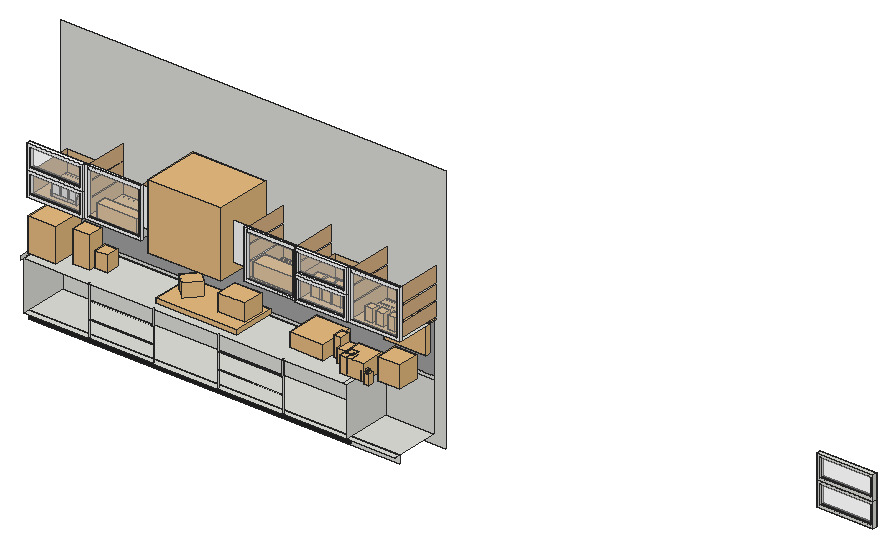
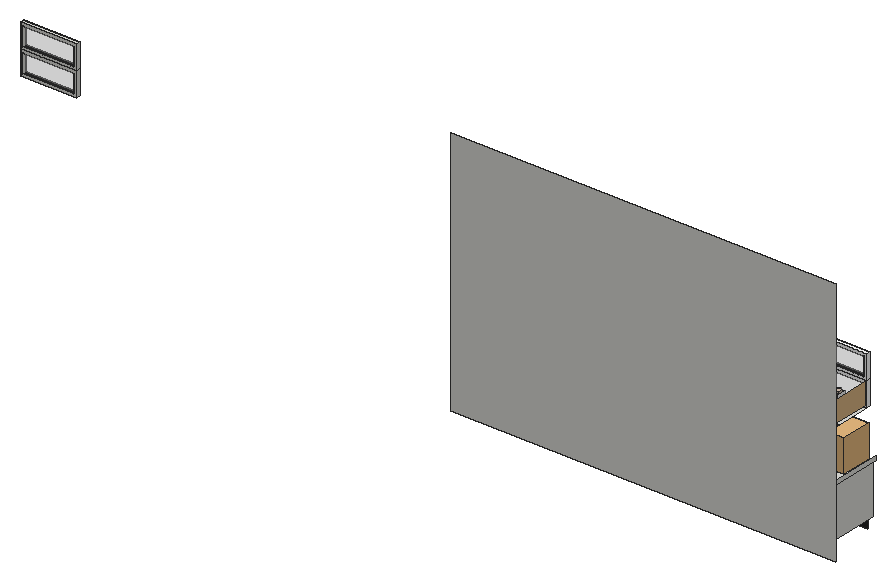
# SketchUp Ruby script. Lengths in inches.
U = 1.inch
M = Sketchup.active_model
def pt(a) = Geom::Point3d.new(a.map { |v| v * U })
def face(e, loops, mat)
  f = e.add_face(loops[0].map { |a| pt(a) })
  loops[1..].each { |l| e.add_face(l.map { |a| pt(a) }).erase! }
  f.material = f.back_material = mat if mat
  f
end
# faces: each face lists its corners as indices into pts; further lists are holes
def faces(e, pts, list, mat = nil) = list.each { |f| face(e, (f[0].is_a?(Array) ? f : [f]).map { |l| l.map { |i| pts[i] } }, mat) }
# xy, xz, yz: faces in a plane at the given z, y or x. An outline is a flat list of corners, or four numbers for a rectangle; further outlines are holes
def ring(l) = l.size == 4 ? [[l[0], l[1]], [l[2], l[1]], [l[2], l[3]], [l[0], l[3]]] : l.each_slice(2).to_a
def flat(e, list, mat, &to3) = list.each { |f| face(e, (f[0].is_a?(Array) ? f : [f]).map { |l| ring(l).map { |u, v| to3.(u, v) } }, mat) }
def xy(e, z, list, mat = nil) = flat(e, list, mat) { |x, y| [x, y, z] }
def xz(e, y, list, mat = nil) = flat(e, list, mat) { |x, z| [x, y, z] }
def yz(e, x, list, mat = nil) = flat(e, list, mat) { |y, z| [x, y, z] }
def lines(e, pts, list) = list.each { |a, b| e.add_line(pt(pts[a]), pt(pts[b])) }
# prism: a flat outline (further loops are holes) pulled along v
def prism(e, loops, v, mat = nil)
  f = face(e, loops, mat); d = Geom::Vector3d.new(v.map { |x| x * U })
  f.pushpull(f.normal.samedirection?(d) ? d.length : -d.length)
end
def box(e, o, s, mat = nil) = prism(e, [[o, [o[0] + s[0], o[1], o[2]], [o[0] + s[0], o[1] + s[1], o[2]], [o[0], o[1] + s[1], o[2]]]], [0, 0, s[2]], mat)
def at(x, y, z, deg = 0) = Geom::Transformation.translation(pt([x, y, z])) * Geom::Transformation.rotation(ORIGIN, Z_AXIS, deg.degrees)
def axes(o, x, y, z) = Geom::Transformation.new([*x, 0, *y, 0, *z, 0, *pt(o).to_a, 1])
def part(name) = M.definitions.add(name)
# library, detail: a bought-in or finely detailed component or shape, given as its bounding box
def library(name, o, s) = part(name).tap { |d| box(d.entities, o, s) }
def detail(e, o, s) = box(e.add_group.entities, o, s)
def put(e, d, t, mat = nil) = e.add_instance(d, t).tap { |i| i.material = mat if mat }
def group(e, t, mat = nil) = e.add_group.tap { |g| g.transformation = t; g.material = mat if mat }.entities
root = M.entities
M.materials.add("Branco").color = [247, 247, 247]
M.materials.add("Etiqueta").color = [244, 244, 244]
M.materials.add("Generic").color = [255, 255, 255]
M.materials.add("Madeira").color = [213, 194, 177]
M.materials.add("[0036_BurlyWood]").color = [222, 184, 135]
M.materials.add("[0136_Charcoal]").color = [35, 35, 35]
M.materials.add("[Mirror 02]").color = [229, 229, 229]
M.materials["[Mirror 02]"].alpha = 0.43
M.materials.add("[Mirror 02]1").color = [229, 229, 229]
M.materials["[Mirror 02]1"].alpha = 0.36
M.materials.add("[Tile Grey]").color = [163, 163, 163]
M.materials.add("cnwhc.com_草图联盟_1kmauOsh").color = [54, 52, 52]
M.materials.add("cnwhc.com_草图联盟_C8Y5Xp2O").color = [156, 156, 156]
M.materials["cnwhc.com_草图联盟_C8Y5Xp2O"].alpha = 0.15
M.materials.add("cnwhc.com_草图联盟_IHFcDxe1").color = [138, 151, 59]
M.materials.add("cnwhc.com_草图联盟_KNEfX85g").color = [162, 126, 87]
M.materials.add("cnwhc.com_草图联盟_QJow1Ky4").color = [144, 133, 65]
M.materials.add("cnwhc.com_草图联盟_z6N5x4Hv").color = [223, 205, 124]
c1 = part("Group\#1")
xy(c1.entities,0,[[0,0,27.625,1.875]])
xy(c1.entities,1.4,[[1.4,0,26.22,0.9375],[1.4,0.9375,26.22,1.875]])
xy(c1.entities,10.58,[[1.4,0,26.22,0.9375],[1.4,0.9375,26.22,1.875]])
xy(c1.entities,11.98,[[0,0,27.625,1.875]])
xy(c1.entities,13.38,[[1.4,0,26.22,0.9375],[1.4,0.9375,26.22,1.875]])
xy(c1.entities,22.56,[[1.4,0,26.22,0.9375],[1.4,0.9375,26.22,1.875]])
xy(c1.entities,23.96,[[0,0,27.625,1.875]])
xz(c1.entities,0,[[[0,0,27.625,11.98],[1.4,1.4,26.22,10.58]],[[0,11.98,27.625,23.96],[1.4,13.38,26.22,22.56]]])
xz(c1.entities,0.9375,[[1.4,1.4,26.22,10.58],[1.4,13.38,26.22,22.56]],"[Mirror 02]")
xz(c1.entities,1.875,[[[0,0,27.625,11.98],[1.4,1.4,26.22,10.58]],[[0,11.98,27.625,23.96],[1.4,13.38,26.22,22.56]]])
yz(c1.entities,0,[[0,0,1.875,11.98],[0,11.98,1.875,23.96]])
yz(c1.entities,1.4,[[0,1.4,0.9375,10.58],[0.9375,1.4,1.875,10.58],[0,13.38,0.9375,22.56],[0.9375,13.38,1.875,22.56]])
yz(c1.entities,26.22,[[0,1.4,0.9375,10.58],[0.9375,1.4,1.875,10.58],[0,13.38,0.9375,22.56],[0.9375,13.38,1.875,22.56]])
yz(c1.entities,27.625,[[0,0,1.875,11.98],[0,11.98,1.875,23.96]])
c2 = part("Group\#107")
xy(c2.entities,0,[[0,0,25.65,1.1875]])
xy(c2.entities,1.23,[[1.61,0,24.42,1.1875]])
xy(c2.entities,22.36,[[1.62,0,24.42,0.59],[1.62,0.59,24.42,1.1875]])
xy(c2.entities,23.17,[[1.61,0,1.62,1.1875]])
xy(c2.entities,23.96,[[0,0,1.62,1.1875],[1.62,0,25.65,1.1875]])
xz(c2.entities,0,[[[0,0,25.65,23.96],[1.61,1.23,1.61,23.17,1.62,23.17,1.62,22.36,24.42,22.36,24.42,1.23]]])
xz(c2.entities,0.59,[[1.62,1.23,24.42,22.36]],"[Mirror 02]1")
xz(c2.entities,1.1875,[[[0,0,25.65,23.96],[1.61,1.23,24.42,1.23,24.42,22.36,1.62,22.36,1.62,23.17,1.61,23.17]]])
yz(c2.entities,0,[[0,0,1.1875,23.96]])
yz(c2.entities,1.61,[[0,1.23,1.1875,23.17]])
yz(c2.entities,1.62,[[0,22.36,1.1875,23.17]])
yz(c2.entities,24.42,[[0,1.23,0.59,22.36],[0.59,1.23,1.1875,22.36]])
yz(c2.entities,25.65,[[0,0,1.1875,23.96]])
c3 = library("Food+jars",[176.18,154.2,55.15],[6.14,23.65,7.76])
c4 = library("Group\#101",[-453.95,-270.9,-0.08],[243.89,243.63,216.82])
c5 = library("Group\#80",[118.34,-437.05,68.8],[33.09,42.97,27.32])
c6 = library("Group\#82",[91.875,-459.8125,1.36],[84.84,84.82,167.94])
c7 = library("Group\#83",[93.63,-458.06,3.28],[81.33,81.31,90.04])
c8 = library("Group\#84",[114.46,-437.1875,150.05],[39.68,39.57,39.67])
c9 = library("Group\#85",[177.52,-496.26,3.28],[81.21,81.23,127.94])
c10 = library("Group\#86",[175.77,-498.01,1.36],[84.71,84.74,167.94])
c11 = library("Group\#87",[198.24,-475.92,149.53],[39.78,40.55,40.71])
c12 = library("Group\#88",[-248.47,-468.28,0.39],[392.05,393.05,278.56])
c13 = library("Group\#89",[-141.57,-278.65,11.2],[96.36,96.33,131.41])
c14 = library("Group\#90",[-62.08,-202.43,11.2],[96.04,96.07,131.41])
c15 = library("Group\#91",[18.13,-280.93,11.2],[96.51,96.54,131.41])
c16 = library("Group\#92",[-213.25,-366.61,11.2],[96.18,96.15,131.41])
c17 = library("Group\#93",[-61.03,-358.93,11.2],[96.54,96.51,131.41])
c18 = library("Group\#94",[8.05,-292.87,22.71],[116.19,111.01,218.49])
c19 = library("Group\#95",[-64.85,-368.89,23],[127.95,108.9,222.0625])
c20 = library("Group\#96",[-143.92,-281.53,22.82],[119.68,105.06,218.38])
c21 = library("Group\#97",[-64.19,-232.55,22.9],[102.65,128.29,224.14])
c22 = library("Group\#98",[-225.25,-376.69,19.19],[116.52,116.69,261.73])
c23 = library("Group\#99",[-138.35,-437.94,11.2],[96.49,96.52,131.41])
c24 = library("Group\#100",[-142.58,-458.38,19.87],[79.66,135.74,256])
c25 = part("KITCHEN+ITEMS+(37)")
put(c25.entities,c4,at(0,0,0))
put(c25.entities,c5,at(0,0,0),"cnwhc.com_草图联盟_IHFcDxe1")
put(c25.entities,c6,at(0,0,0),"cnwhc.com_草图联盟_C8Y5Xp2O")
put(c25.entities,c7,at(0,0,0),"cnwhc.com_草图联盟_QJow1Ky4")
put(c25.entities,c8,at(0,0,0),"cnwhc.com_草图联盟_KNEfX85g")
put(c25.entities,c9,at(0,0,0),"cnwhc.com_草图联盟_z6N5x4Hv")
put(c25.entities,c10,at(0,0,0),"cnwhc.com_草图联盟_C8Y5Xp2O")
put(c25.entities,c11,at(0,0,0),"cnwhc.com_草图联盟_KNEfX85g")
put(c25.entities,c12,at(0,0,0),"cnwhc.com_草图联盟_1kmauOsh")
put(c25.entities,c13,at(0,0,0),"cnwhc.com_草图联盟_C8Y5Xp2O")
put(c25.entities,c14,at(0,0,0),"cnwhc.com_草图联盟_C8Y5Xp2O")
put(c25.entities,c15,at(0,0,0),"cnwhc.com_草图联盟_C8Y5Xp2O")
put(c25.entities,c16,at(0,0,0),"cnwhc.com_草图联盟_C8Y5Xp2O")
put(c25.entities,c17,at(0,0,0),"cnwhc.com_草图联盟_C8Y5Xp2O")
put(c25.entities,c18,at(0,0,0),"cnwhc.com_草图联盟_1kmauOsh")
put(c25.entities,c19,at(0,0,0),"cnwhc.com_草图联盟_1kmauOsh")
put(c25.entities,c20,at(0,0,0),"cnwhc.com_草图联盟_1kmauOsh")
put(c25.entities,c21,at(0,0,0),"cnwhc.com_草图联盟_1kmauOsh")
put(c25.entities,c22,at(0,0,0))
put(c25.entities,c23,at(0,0,0),"cnwhc.com_草图联盟_C8Y5Xp2O")
put(c25.entities,c24,at(0,0,0))
c26 = library("Group\#6",[-374.05,84.21,613.65],[72.44,72.44,111.8])
c27 = library("Group\#5",[-462.66,84.21,613.65],[72.44,72.44,111.8])
c28 = library("Group\#7",[-289.4,84.22,613.65],[72.44,72.43,111.8])
c29 = library("Potted plant pair",[-0.125,-0.11,0],[4.84,5.4,5.74])
c30 = library("mixer",[2.53,2.84,0],[8.2,7.51,15.59])
c31 = library("Kitchenware display",[-1.93,-1.45,-0.01],[13.28,36.8,12.14])
c32 = part("Agrupar\#12")
xy(c32.entities,0,[[-280.31,0,-272.11,0.79],[0,0,0,0.79,-280.31,0.79,-280.31,161.02,0,161.02,0,161.8125,10.17,161.8125,10.17,0],[-280.31,161.02,-272.11,161.8125]],"Madeira")
xy(c32.entities,11.05,[[-272.11,11.05,0,150.76]],"Madeira")
xy(c32.entities,41.2,[[-272.11,0.79,0,11.05]],"Madeira")
xy(c32.entities,69.3,[[-272.11,150.76,0,161.02]],"Madeira")
xy(c32.entities,76.35,[[-280.31,0,-272.11,26.97],[0,0,10.17,26.97],[-280.31,134.84,-272.11,161.8125],[0,134.84,10.17,161.8125]],"Madeira")
xz(c32.entities,0,[[-280.31,0,-272.11,76.35],[0,0,10.17,76.35]],"Madeira")
xz(c32.entities,0.79,[[-272.11,0,0,41.2]],"Madeira")
xz(c32.entities,11.05,[[-272.11,11.05,0,41.2]],"Madeira")
xz(c32.entities,150.76,[[-272.11,11.05,0,69.3]],"Madeira")
xz(c32.entities,161.02,[[-272.11,0,0,69.3]],"Madeira")
xz(c32.entities,161.8125,[[-280.31,0,-272.11,76.35],[0,0,10.17,76.35]],"Madeira")
yz(c32.entities,-280.31,[[[0,0,0,76.35,26.97,76.35,31.83,88.93,32.51,90.6875,39.09,100.58,47.67,108.82,57.83,115,69.09,118.82,80.91,120.12,92.72,118.82,103.98,115,114.14,108.82,122.72,100.58,129.3,90.6875,129.98,88.93,134.84,76.35,161.8125,76.35,161.8125,0],[80.91,27.05,93.61,28.72,105.44,33.625,115.61,41.42,123.41,51.59,125.76,57.26,125.79,57.33,127.05,60.38,126.3,62.19,123.53,68.87,123.41,69.17,115.61,79.33,105.44,87.13,93.61,92.04,80.91,93.71,68.2,92.04,56.37,87.13,46.2,79.33,38.4,69.17,38.28,68.87,35.51,62.19,34.76,60.38,36.02,57.33,36.05,57.26,38.4,51.59,46.2,41.42,56.37,33.625,68.2,28.72]]],"Madeira")
yz(c32.entities,-272.11,[[[0,0,0.79,0,0.79,41.2,11.05,41.2,11.05,11.05,150.76,11.05,150.76,69.3,161.02,69.3,161.02,0,161.8125,0,161.8125,76.35,134.84,76.35,129.98,88.93,129.3,90.6875,122.72,100.58,114.14,108.82,103.98,115,92.72,118.82,80.91,120.12,69.09,118.82,57.83,115,47.67,108.82,39.09,100.58,32.51,90.6875,31.83,88.93,26.97,76.35,0,76.35],[80.91,27.05,68.2,28.72,56.37,33.625,46.2,41.42,38.4,51.59,36.05,57.26,36.02,57.33,34.76,60.38,35.51,62.19,38.28,68.87,38.4,69.17,46.2,79.33,56.37,87.13,68.2,92.04,80.91,93.71,93.61,92.04,105.44,87.13,115.61,79.33,123.41,69.17,123.53,68.87,126.3,62.19,127.05,60.38,125.79,57.33,125.76,57.26,123.41,51.59,115.61,41.42,105.44,33.625,93.61,28.72]]],"Madeira")
yz(c32.entities,0,[[[0,0,0,76.35,26.97,76.35,31.83,88.93,32.51,90.6875,39.09,100.58,47.67,108.82,57.83,115,69.09,118.82,80.91,120.12,92.72,118.82,103.98,115,114.14,108.82,122.72,100.58,129.3,90.6875,129.98,88.93,134.84,76.35,150.76,76.35,150.76,11.05,11.05,11.05,11.05,41.2,0.79,41.2,0.79,0],[80.91,27.05,93.61,28.72,105.44,33.625,115.61,41.42,123.41,51.59,125.76,57.26,125.79,57.33,127.05,60.38,126.3,62.19,123.53,68.87,123.41,69.17,115.61,79.33,105.44,87.13,93.61,92.04,80.91,93.71,68.2,92.04,56.37,87.13,46.2,79.33,38.4,69.17,38.28,68.87,35.51,62.19,34.76,60.38,36.02,57.33,36.05,57.26,38.4,51.59,46.2,41.42,56.37,33.625,68.2,28.72]],[161.02,0,161.8125,76.35],[150.76,69.3,161.02,76.35]],"Madeira")
yz(c32.entities,10.17,[[[0,0,161.8125,0,161.8125,76.35,134.84,76.35,129.98,88.93,129.3,90.6875,122.72,100.58,114.14,108.82,103.98,115,92.72,118.82,80.91,120.12,69.09,118.82,57.83,115,47.67,108.82,39.09,100.58,32.51,90.6875,31.83,88.93,26.97,76.35,0,76.35],[80.91,27.05,68.2,28.72,56.37,33.625,46.2,41.42,38.4,51.59,36.05,57.26,36.02,57.33,34.76,60.38,35.51,62.19,38.28,68.87,38.4,69.17,46.2,79.33,56.37,87.13,68.2,92.04,80.91,93.71,93.61,92.04,105.44,87.13,115.61,79.33,123.41,69.17,123.53,68.87,126.3,62.19,127.05,60.38,125.79,57.33,125.76,57.26,123.41,51.59,115.61,41.42,105.44,33.625,93.61,28.72]]],"Madeira")
p = [[-280.31,80.91,27.05],[-280.31,68.2,28.72],[-272.11,68.2,28.72],[-272.11,80.91,27.05],[10.17,68.2,28.72],[10.17,80.91,27.05],
  [0,80.91,27.05],[0,68.2,28.72],[-280.31,93.61,28.72],[-272.11,93.61,28.72],[10.17,93.61,28.72],[0,93.61,28.72],
  [-280.31,56.37,33.625],[-272.11,56.37,33.625],[10.17,56.37,33.625],[0,56.37,33.625],[-280.31,105.44,33.625],[-272.11,105.44,33.625],
  [10.17,105.44,33.625],[0,105.44,33.625],[-280.31,46.2,41.42],[-272.11,46.2,41.42],[10.17,46.2,41.42],[0,46.2,41.42],
  [-280.31,115.61,41.42],[-272.11,115.61,41.42],[10.17,115.61,41.42],[0,115.61,41.42],[-280.31,38.4,51.59],[-272.11,38.4,51.59],
  [10.17,38.4,51.59],[0,38.4,51.59],[-280.31,123.41,51.59],[-272.11,123.41,51.59],[10.17,123.41,51.59],[0,123.41,51.59],
  [-280.31,36.05,57.26],[-272.11,36.05,57.26],[10.17,36.05,57.26],[0,36.05,57.26],[-280.31,125.76,57.26],[-272.11,125.76,57.26],
  [10.17,125.76,57.26],[0,125.76,57.26],[-280.31,36.02,57.33],[-280.31,34.76,60.38],[-272.11,34.76,60.38],[-272.11,36.02,57.33],
  [10.17,34.76,60.38],[10.17,36.02,57.33],[0,36.02,57.33],[0,34.76,60.38],[-280.31,125.79,57.33],[-272.11,125.79,57.33],
  [-280.31,127.05,60.38],[-272.11,127.05,60.38],[10.17,125.79,57.33],[0,125.79,57.33],[10.17,127.05,60.38],[0,127.05,60.38],
  [-280.31,35.51,62.19],[-272.11,35.51,62.19],[10.17,35.51,62.19],[0,35.51,62.19],[-280.31,126.3,62.19],[-272.11,126.3,62.19],
  [10.17,126.3,62.19],[0,126.3,62.19],[-280.31,38.28,68.87],[-272.11,38.28,68.87],[10.17,38.28,68.87],[0,38.28,68.87],
  [-280.31,123.53,68.87],[-272.11,123.53,68.87],[10.17,123.53,68.87],[0,123.53,68.87],[-280.31,38.4,69.17],[-272.11,38.4,69.17],
  [10.17,38.4,69.17],[0,38.4,69.17],[-280.31,123.41,69.17],[-272.11,123.41,69.17],[10.17,123.41,69.17],[0,123.41,69.17],
  [-280.31,46.2,79.33],[-272.11,46.2,79.33],[10.17,46.2,79.33],[0,46.2,79.33],[-280.31,115.61,79.33],[-272.11,115.61,79.33],
  [10.17,115.61,79.33],[0,115.61,79.33],[-280.31,31.83,88.93],[-280.31,26.97,76.35],[-272.11,26.97,76.35],[-272.11,31.83,88.93],
  [10.17,26.97,76.35],[10.17,31.83,88.93],[0,31.83,88.93],[0,26.97,76.35],[-280.31,134.84,76.35],[-280.31,129.98,88.93],
  [-272.11,129.98,88.93],[-272.11,134.84,76.35],[10.17,129.98,88.93],[10.17,134.84,76.35],[0,134.84,76.35],[0,129.98,88.93],
  [-280.31,56.37,87.13],[-272.11,56.37,87.13],[10.17,56.37,87.13],[0,56.37,87.13],[-280.31,105.44,87.13],[-272.11,105.44,87.13],
  [10.17,105.44,87.13],[0,105.44,87.13],[-280.31,68.2,92.04],[-272.11,68.2,92.04],[10.17,68.2,92.04],[0,68.2,92.04],
  [-280.31,93.61,92.04],[-272.11,93.61,92.04],[10.17,93.61,92.04],[0,93.61,92.04],[-280.31,32.51,90.6875],[-272.11,32.51,90.6875],
  [10.17,32.51,90.6875],[0,32.51,90.6875],[-280.31,129.3,90.6875],[-272.11,129.3,90.6875],[10.17,129.3,90.6875],[0,129.3,90.6875],
  [-280.31,39.09,100.58],[-272.11,39.09,100.58],[10.17,39.09,100.58],[0,39.09,100.58],[-280.31,122.72,100.58],[-272.11,122.72,100.58],
  [10.17,122.72,100.58],[0,122.72,100.58],[-280.31,80.91,93.71],[-272.11,80.91,93.71],[10.17,80.91,93.71],[0,80.91,93.71],
  [-280.31,47.67,108.82],[-272.11,47.67,108.82],[10.17,47.67,108.82],[0,47.67,108.82],[-280.31,114.14,108.82],[-272.11,114.14,108.82],
  [10.17,114.14,108.82],[0,114.14,108.82],[-280.31,57.83,115],[-272.11,57.83,115],[10.17,57.83,115],[0,57.83,115],
  [-280.31,103.98,115],[-272.11,103.98,115],[10.17,103.98,115],[0,103.98,115],[-280.31,69.09,118.82],[-272.11,69.09,118.82],
  [10.17,69.09,118.82],[0,69.09,118.82],[-280.31,92.72,118.82],[-272.11,92.72,118.82],[10.17,92.72,118.82],[0,92.72,118.82],
  [-280.31,80.91,120.12],[-272.11,80.91,120.12],[10.17,80.91,120.12],[0,80.91,120.12],[-272.11,150.76,11.05],[-272.11,150.76,0],
  [-272.11,11.05,11.05],[-272.11,11.05,0]]
faces(c32.entities,p,[[0,1,2,3],[4,5,6,7],[8,0,3,9],[5,10,11,6],[1,12,13,2],[14,4,7,15],[16,8,9,17],[10,18,19,11],
  [12,20,21,13],[22,14,15,23],[24,16,17,25],[18,26,27,19],[20,28,29,21],[30,22,23,31],[32,24,25,33],[26,34,35,27],
  [28,36,37,29],[38,30,31,39],[40,32,33,41],[34,42,43,35],[44,45,46,47],[48,49,50,51],[36,44,47,37],[49,38,39,50],
  [52,40,41,53],[54,52,53,55],[42,56,57,43],[56,58,59,57],[45,60,61,46],[62,48,51,63],[64,54,55,65],[58,66,67,59],
  [60,68,69,61],[70,62,63,71],[72,64,65,73],[66,74,75,67],[68,76,77,69],[78,70,71,79],[80,72,73,81],[74,82,83,75],
  [76,84,85,77],[86,78,79,87],[88,80,81,89],[82,90,91,83],[92,93,94,95],[96,97,98,99],[100,101,102,103],[104,105,106,107],
  [84,108,109,85],[110,86,87,111],[112,88,89,113],[90,114,115,91],[108,116,117,109],[118,110,111,119],[120,112,113,121],[114,122,123,115],
  [124,92,95,125],[97,126,127,98],[101,128,129,102],[130,104,107,131],[132,124,125,133],[126,134,135,127],[128,136,137,129],[138,130,131,139],
  [116,140,141,117],[142,118,119,143],[140,120,121,141],[122,142,143,123],[144,132,133,145],[134,146,147,135],[136,148,149,137],[150,138,139,151],
  [152,144,145,153],[146,154,155,147],[148,156,157,149],[158,150,151,159],[160,152,153,161],[154,162,163,155],[156,164,165,157],[166,158,159,167],
  [168,160,161,169],[162,170,171,163],[164,168,169,165],[170,166,167,171]],"Madeira")
lines(c32.entities,p,[[172,173],[174,175]])
c33 = part("Agrupar\#11")
xy(c33.entities,0,[[0,0,86.61,89.37]],"Branco")
xy(c33.entities,123.62,[[[0,0,86.61,89.37],[43.18,1.77,6.08,23.34,6.14,44.69,6.21,66.25,43.31,87.52,43.43,87.6,80.53,66.03,80.47,44.69,80.41,23.12,43.31,1.85]]],"Branco")
xy(c33.entities,138.1875,[[43.18,1.77,43.31,1.85,80.41,23.12,80.47,44.69,80.53,66.03,43.43,87.6,43.31,87.52,6.21,66.25,6.14,44.69,6.08,23.34]],"Madeira")
xz(c33.entities,0,[[0,0,86.61,123.62]],"Etiqueta")
xz(c33.entities,89.37,[[0,0,86.61,123.62]],"Branco")
yz(c33.entities,0,[[0,0,89.37,123.62]],"Branco")
yz(c33.entities,86.61,[[0,0,89.37,123.62]],"Branco")
p = [[6.08,23.34,123.62],[43.18,1.77,123.62],[43.18,1.77,138.1875],[6.08,23.34,138.1875],[43.31,1.85,123.62],[80.41,23.12,123.62],
  [80.41,23.12,138.1875],[43.31,1.85,138.1875],[80.47,44.69,123.62],[80.53,66.03,123.62],[80.53,66.03,138.1875],[80.47,44.69,138.1875],
  [6.21,66.25,123.62],[6.14,44.69,123.62],[6.14,44.69,138.1875],[6.21,66.25,138.1875],[43.43,87.6,123.62],[43.43,87.6,138.1875],
  [43.31,87.52,123.62],[43.31,87.52,138.1875]]
faces(c33.entities,p,[[0,1,2,3],[1,4,5,6,7,2],[5,8,9,10,11,6],[12,13,0,3,14,15],[9,16,17,10],[16,18,12,15,19,17]],"Madeira")
c34 = part("Agrupar\#10")
xy(c34.entities,0,[[0,0,86.61,89.37]],"Branco")
xy(c34.entities,123.62,[[[0,0,86.61,89.37],[43.18,1.77,6.08,23.34,6.14,44.69,6.21,66.25,43.31,87.52,43.43,87.6,80.53,66.03,80.47,44.69,80.41,23.12,43.31,1.85]]],"Branco")
xy(c34.entities,138.1875,[[43.18,1.77,43.31,1.85,80.41,23.12,80.47,44.69,80.53,66.03,43.43,87.6,43.31,87.52,6.21,66.25,6.14,44.69,6.08,23.34]],"Madeira")
xz(c34.entities,0,[[0,0,86.61,123.62]],"Etiqueta")
xz(c34.entities,89.37,[[0,0,86.61,123.62]],"Branco")
yz(c34.entities,0,[[0,0,89.37,123.62]],"Branco")
yz(c34.entities,86.61,[[0,0,89.37,123.62]],"Branco")
p = [[6.08,23.34,123.62],[43.18,1.77,123.62],[43.18,1.77,138.1875],[6.08,23.34,138.1875],[43.31,1.85,123.62],[80.41,23.12,123.62],
  [80.41,23.12,138.1875],[43.31,1.85,138.1875],[80.47,44.69,123.62],[80.53,66.03,123.62],[80.53,66.03,138.1875],[80.47,44.69,138.1875],
  [6.21,66.25,123.62],[6.14,44.69,123.62],[6.14,44.69,138.1875],[6.21,66.25,138.1875],[43.43,87.6,123.62],[43.43,87.6,138.1875],
  [43.31,87.52,123.62],[43.31,87.52,138.1875]]
faces(c34.entities,p,[[0,1,2,3],[1,4,5,6,7,2],[5,8,9,10,11,6],[12,13,0,3,14,15],[9,16,17,10],[16,18,12,15,19,17]],"Madeira")
c35 = part("Agrupar\#9")
xy(c35.entities,0,[[0,0,86.61,89.37]],"Branco")
xy(c35.entities,123.62,[[[0,0,86.61,89.37],[43.18,1.77,6.08,23.34,6.14,44.69,6.21,66.25,43.31,87.52,43.43,87.6,80.53,66.03,80.47,44.69,80.41,23.12,43.31,1.85]]],"Branco")
xy(c35.entities,138.1875,[[43.18,1.77,43.31,1.85,80.41,23.12,80.47,44.69,80.53,66.03,43.43,87.6,43.31,87.52,6.21,66.25,6.14,44.69,6.08,23.34]],"Madeira")
xz(c35.entities,0,[[0,0,86.61,123.62]],"Etiqueta")
xz(c35.entities,89.37,[[0,0,86.61,123.62]],"Branco")
yz(c35.entities,0,[[0,0,89.37,123.62]],"Branco")
yz(c35.entities,86.61,[[0,0,89.37,123.62]],"Branco")
p = [[6.08,23.34,123.62],[43.18,1.77,123.62],[43.18,1.77,138.1875],[6.08,23.34,138.1875],[43.31,1.85,123.62],[80.41,23.12,123.62],
  [80.41,23.12,138.1875],[43.31,1.85,138.1875],[80.47,44.69,123.62],[80.53,66.03,123.62],[80.53,66.03,138.1875],[80.47,44.69,138.1875],
  [6.21,66.25,123.62],[6.14,44.69,123.62],[6.14,44.69,138.1875],[6.21,66.25,138.1875],[43.43,87.6,123.62],[43.43,87.6,138.1875],
  [43.31,87.52,123.62],[43.31,87.52,138.1875]]
faces(c35.entities,p,[[0,1,2,3],[1,4,5,6,7,2],[5,8,9,10,11,6],[12,13,0,3,14,15],[9,16,17,10],[16,18,12,15,19,17]],"Madeira")
c36 = part("TDS")
put(c36.entities,c32,axes([280.31,0,0],[1,0,0],[0,0.66912,0],[0,0,0.67]))
put(c36.entities,c33,at(191.09,9.47,11.02))
put(c36.entities,c34,at(100.9375,9.47,11.02))
put(c36.entities,c35,at(9.6,9.47,11.02))
c37 = part("jar")
put(c37.entities,c36,at(-649.15,-679.88,0))
c38 = library("PV977NSS_GEProfile",[-17.9375,-27.5625,-0.25],[35.95,27.64,32.08])
c39 = library("Group\#16",[-198.8,84.74,613.85],[84,84,172.39])
c40 = library("Group\#18",[-15.73,84.74,613.85],[84,84,172.39])
c41 = library("Group\#17",[-105.26,84.74,613.85],[84,84,172.39])
c42 = library("Stacked bowls",[0,0,0],[8.98,8.99,10.96])
c43 = library("C_HOB",[0,0,0],[30.71,17.32,2.28])
c44 = library("PLATE",[-1.81,0,33.86],[10.25,10.83,10.53])
c45 = library("pot (1)",[31.4375,7.2,0.01],[13.32,10.03,8.54])
c46 = library("FORK+&+SPOON",[7.6,1.73,0],[3.73,4.8,9.78])
c47 = library("飛利浦電熱壺+(SU+2018)",[-0.68,-0.52,0],[10.49,12.89,12.43])
c48 = library("vm_v2_031",[-4.73,-4.73,0],[9.46,9.46,3.85])
c49 = library("Kitchen Utensil.",[-24.86,-2.29,-26.5],[81.83,11.85,18.87])
c50 = library("Group\#49",[-0.5,-0.5,-0.1],[77.94,3.6875,0.2])
c51 = library("Group\#48",[-0.5,-0.5,-0.1],[56.25,3.1875,0.2])
c52 = library("skpC936",[0,-1.9,0],[21.12,3.04,12.85])
xy(root,6.5625,[[7.99,403.75,7.99,406.75,167,406.75,167,403.75,135.5,403.75,135.5,404.32,135.2,404.32,135.2,403.75,103.69,403.75,103.69,404.32,103.39,404.32,103.39,403.75,71.89,403.75,71.89,404.32,71.59,404.32,71.59,403.75,40.09,403.75,40.09,404.32,39.79,404.32,39.79,403.75],[167,403.75,190.94,406.75],[190.94,403.75,191,406.75],[7.99,406.75,167,427.75],[167,406.75,190.94,427.75],
  [190.94,406.75,191,427.75]])
xy(root,30.5625,[[7.99,403.75,7.99,427.75,165,427.75,165,403.75,135.5,403.75,135.5,404.32,135.2,404.32,135.2,403.75,103.69,403.75,103.69,404.32,103.39,404.32,103.39,403.75,71.89,403.75,71.89,404.32,71.59,404.32,71.59,403.75,40.09,403.75,40.09,404.32,39.79,404.32,39.79,403.75],[165,403.75,167,427.75]])
xy(root,56.6,[[7.99,407.75,63.24,425.57],[114.06,407.75,191,425.07]])
xy(root,57.38,[[8.77,407.75,34.84,429.57],[36.39,407.75,62.46,429.57]],"[0036_BurlyWood]")
xy(root,57.39,[[114.85,407.75,138.91,429.57],[140.5,407.75,164.56,429.57],[166.14,407.75,190.2,429.57]],"[0036_BurlyWood]")
xy(root,62.1,[[63.24,407.75,114.06,427.75]])
xz(root,404.32,[[39.79,6.5625,40.09,30.5625],[71.59,6.5625,71.89,30.5625],[103.39,6.5625,103.69,30.5625],[135.2,6.5625,135.5,30.5625],[40.09,14.5625,71.59,14.86],
  [103.69,14.5625,135.2,14.86],[40.09,22.5625,71.59,22.86],[103.69,22.5625,135.2,22.86]])
xz(root,406.75,[[167,2.5625,191,6.5625]])
xz(root,406.75,[[7.99,2.5625,167,6.5625]],"[0136_Charcoal]")
xz(root,407.75,[[[7.99,56.6,35.61,68.58],[8.77,57.38,34.84,67.8]],[[35.61,56.6,63.24,80.5625],[36.39,57.38,62.46,79.79]],[[114.06,56.6,139.7,80.5625],[114.85,57.39,138.91,79.77]],[[139.7,56.6,165.35,80.5625],[140.5,57.39,164.56,79.77]],[[165.35,56.6,191,80.5625],[166.14,57.39,190.2,79.77]]])
xz(root,407.75,[[63.24,62.1,114.06,80.5625]],"Generic")
xz(root,425.07,[[114.06,56.6,191,57.16]])
xz(root,425.57,[[7.99,56.6,63.24,56.97]])
xz(root,427.75,[[7.99,6.5625,167,30.5625],[167,6.5625,190.94,30.5625],[190.94,6.5625,191,30.5625],[7.99,30.5625,165,32.5625],[165,30.5625,167,32.5625],
  [167,30.5625,191,32.5625]])
xz(root,427.75,[[7.99,32.5625,191,32.5625,191,57.16,114.06,57.16,114.06,62.1,63.24,62.1,63.24,56.97,7.99,56.97]],"[Tile Grey]")
xz(root,429.57,[[8.77,57.38,34.84,67.8],[36.39,57.38,62.46,64.03],[114.85,57.39,138.91,64.04],[140.5,57.39,164.56,67.74],[166.14,57.39,190.2,63.79]],"[0036_BurlyWood]")
xz(root,431,[[4.74,0,194.24,122.5625]])
yz(root,7.99,[[403.75,6.5625,427.75,30.5625],[401.75,30.5625,427.75,32.5625]])
yz(root,8.77,[[407.75,57.38,429.57,67.8]],"[0036_BurlyWood]")
yz(root,34.84,[[407.75,57.38,429.57,67.8]],"[0036_BurlyWood]")
yz(root,36.39,[[407.75,57.38,429.57,57.38,429.57,64.03,410.57,64.03,410.57,64.85,429.57,64.85,429.57,71.5,410.57,71.5,410.57,72.32,429.57,72.32,429.57,79.79,407.75,79.79]],"[0036_BurlyWood]")
yz(root,62.46,[[407.75,57.38,407.75,79.79,429.57,79.79,429.57,72.32,410.57,72.32,410.57,71.5,429.57,71.5,429.57,64.85,410.57,64.85,410.57,64.03,429.57,64.03,429.57,57.38]],"[0036_BurlyWood]")
yz(root,63.24,[[407.75,56.6,425.57,56.6,425.57,56.97,427.75,56.97,427.75,62.1,407.75,62.1]])
yz(root,71.59,[[403.75,22.86,404.32,30.5625]])
yz(root,114.06,[[407.75,56.6,407.75,62.1,427.75,62.1,427.75,57.16,425.07,57.16,425.07,56.6]])
yz(root,114.85,[[407.75,57.39,429.57,57.39,429.57,64.04,409.25,64.04,409.25,64.85,429.57,64.85,429.57,71.5,409.25,71.5,409.25,72.3125,429.57,72.3125,429.57,79.77,407.75,79.77]],"[0036_BurlyWood]")
yz(root,135.2,[[403.75,22.86,404.32,30.5625]])
yz(root,138.91,[[407.75,57.39,407.75,79.77,429.57,79.77,429.57,72.3125,409.25,72.3125,409.25,71.5,429.57,71.5,429.57,64.85,409.25,64.85,409.25,64.04,429.57,64.04,429.57,57.39]],"[0036_BurlyWood]")
yz(root,140.5,[[407.75,57.39,429.57,67.74]],"[0036_BurlyWood]")
yz(root,164.56,[[407.75,57.39,429.57,67.74]],"[0036_BurlyWood]")
yz(root,166.14,[[407.75,57.39,429.57,57.39,429.57,63.79,409.25,63.79,409.25,64.85,429.57,64.85,429.57,71.25,409.25,71.25,409.25,72.3125,429.57,72.3125,429.57,79.77,407.75,79.77]],"[0036_BurlyWood]")
yz(root,167,[[403.75,6.5625,427.75,30.5625]])
yz(root,190.2,[[407.75,57.39,407.75,79.77,429.57,79.77,429.57,72.3125,409.25,72.3125,409.25,71.25,429.57,71.25,429.57,64.85,409.25,64.85,409.25,63.79,429.57,63.79,429.57,57.39]],"[0036_BurlyWood]")
put(root,c1,at(397.18,405.88,56.6))
put(root,c1,axes([139.7,405.88,56.6],[0.9288,0,0],[0,1,0],[0,0,1]),"Generic")
put(root,c1,axes([7.77,405.88,56.6],[1.00808,0,0],[0,1,0],[0,0,1]),"Generic")
put(root,c2,at(165.35,406.57,56.6),"Generic")
put(root,c2,at(114.06,406.57,56.6),"Generic")
put(root,c2,axes([35.61,406.57,56.6],[1.09278,0,0],[0,1,0],[0,0,1]),"Generic")
put(root,c3,axes([191.12,258.92,10.5],[0,0.85,0],[-0.85,0,0],[0,0,0.85]))
put(root,c25,axes([168.93,420.375,32.56],[0.02942,0,0],[0,0.02942,0],[0,0,0.02942]))
put(root,c26,axes([195.61,406.34,24.93],[0.05291,0,0],[0,0.05291,0],[0,0,0.05291]))
put(root,c27,axes([195.01,406.34,24.93],[0.05291,0,0],[0,0.05291,0],[0,0,0.05291]))
put(root,c28,axes([196.93,406.34,24.93],[0.05291,0,0],[0,0.05291,0],[0,0,0.05291]))
put(root,c29,axes([9.29,405.73,32.5625],[2.81,0,0],[0,2.81,0],[0,0,2.81]))
put(root,c30,at(25.1875,406.52,32.5625))
put(root,c31,axes([136.05,410.85,57.39],[0,0.56799,0],[-0.56799,0,0],[0,0,0.56799]))
put(root,c37,axes([43.62,441.5,57.38],[0.044,0,0],[0,0.044,0],[0,0,0.044]))
put(root,c38,at(90.03,427.75,57.41))
put(root,c39,axes([152.78,408.27,25.34],[0.0517,0,0],[0,0.0517,0],[0,0,0.0517]))
put(root,c40,axes([153.59,408.27,25.34],[0.0517,0,0],[0,0.0517,0],[0,0,0.0517]))
put(root,c40,axes([158.96,408.27,25.34],[0.0517,0,0],[0,0.0517,0],[0,0,0.0517]))
put(root,c41,axes([153.28,408.27,25.34],[0.0517,0,0],[0,0.0517,0],[0,0,0.0517]))
put(root,c42,axes([36.33,412.39,32.5625],[0.69,0,0],[0,0.69,0],[0,0,0.69]))
put(root,c43,axes([72.02,405.1,32.5625],[1.2992,0,0],[0,1.2,0],[0,0,1]))
put(root,c44,at(176.57,419.65,-1.3,-90))
put(root,c45,at(65.76,404.8,34.62))
put(root,c46,at(144.33,413.06,32.5625))
put(root,c47,axes([84.76,418.09,33.07],[-0.4985,0.44885,0],[-0.44885,-0.4985,0],[0,0,0.6708]))
put(root,c48,axes([142,418.61,32.5625],[1.76,0,0],[0,1.76,0],[0,0,1.76]))
put(root,c49,axes([154.15,426.85,57.35],[-0.3936,0,0],[0,-0.3936,0],[0,0,0.3936]))
put(root,c50,at(114.06,425.07,57.16))
put(root,c51,at(7.99,425.57,56.97))
put(root,c52,at(167.53,427.75,41.36))
